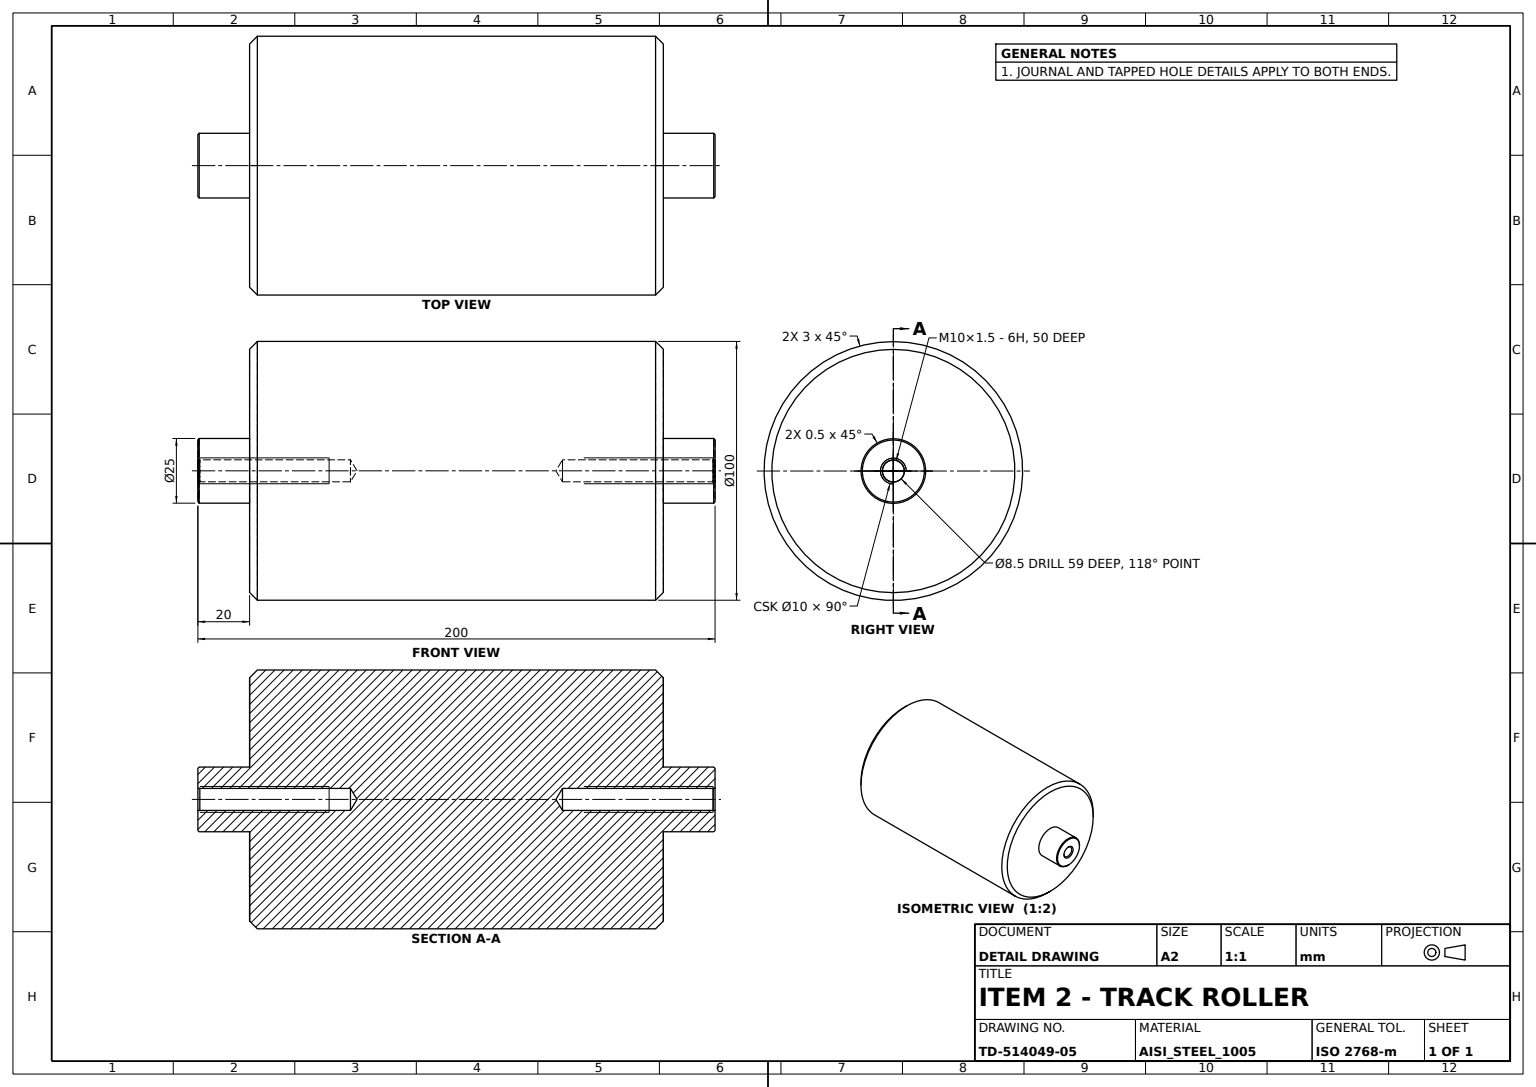
ISO-10303-21;
HEADER;
FILE_DESCRIPTION((''),'2;1');
FILE_NAME('','',(''),(''),'','','');
FILE_SCHEMA(('AUTOMOTIVE_DESIGN'));
ENDSEC;
DATA;
#1=APPLICATION_CONTEXT('');
#2=PRODUCT_CONTEXT('',#1,'mechanical');
#3=PRODUCT('','','',(#2));
#4=PRODUCT_DEFINITION_FORMATION('','',#3);
#5=PRODUCT_DEFINITION_CONTEXT('',#1,'design');
#6=PRODUCT_DEFINITION('','',#4,#5);
#7=PRODUCT_DEFINITION_SHAPE('','',#6);
#8=(LENGTH_UNIT()NAMED_UNIT(*)SI_UNIT(.MILLI.,.METRE.));
#9=(NAMED_UNIT(*)PLANE_ANGLE_UNIT()SI_UNIT($,.RADIAN.));
#10=(NAMED_UNIT(*)SI_UNIT($,.STERADIAN.)SOLID_ANGLE_UNIT());
#11=UNCERTAINTY_MEASURE_WITH_UNIT(LENGTH_MEASURE(0.005),#8,'distance_accuracy_value','');
#12=(GEOMETRIC_REPRESENTATION_CONTEXT(3)GLOBAL_UNCERTAINTY_ASSIGNED_CONTEXT((#11))GLOBAL_UNIT_ASSIGNED_CONTEXT((#8,#9,#10))REPRESENTATION_CONTEXT('',''));
#13=CARTESIAN_POINT('',(-12.,0.,100.));
#14=VERTEX_POINT('',#13);
#15=CARTESIAN_POINT('',(0.,0.,100.));
#16=DIRECTION('',(0.,0.,-1.));
#17=DIRECTION('',(-1.,0.,0.));
#18=AXIS2_PLACEMENT_3D('',#15,#16,#17);
#19=CIRCLE('',#18,12.);
#20=EDGE_CURVE('',#14,#14,#19,.F.);
#21=ORIENTED_EDGE('',*,*,#20,.T.);
#22=EDGE_LOOP('',(#21));
#23=FACE_BOUND('',#22,.T.);
#24=CARTESIAN_POINT('',(-5.,0.,100.));
#25=VERTEX_POINT('',#24);
#26=CIRCLE('',#18,5.);
#27=EDGE_CURVE('',#25,#25,#26,.T.);
#28=ORIENTED_EDGE('',*,*,#27,.T.);
#29=EDGE_LOOP('',(#28));
#30=FACE_BOUND('',#29,.T.);
#31=PLANE('',#18);
#32=ADVANCED_FACE('',(#23,#30),#31,.F.);
#33=CARTESIAN_POINT('',(4.25,0.,-41.));
#34=VERTEX_POINT('',#33);
#35=CARTESIAN_POINT('',(0.,0.,-41.));
#36=DIRECTION('',(0.,0.,1.));
#37=DIRECTION('',(1.,0.,0.));
#38=AXIS2_PLACEMENT_3D('',#35,#36,#37);
#39=CIRCLE('',#38,4.25);
#40=EDGE_CURVE('',#34,#34,#39,.T.);
#41=ORIENTED_EDGE('',*,*,#40,.F.);
#42=EDGE_LOOP('',(#41));
#43=FACE_BOUND('',#42,.T.);
#44=CARTESIAN_POINT('',(0.,0.,-38.446342));
#45=VERTEX_POINT('',#44);
#46=VERTEX_LOOP('',#45);
#47=FACE_BOUND('',#46,.T.);
#48=AXIS2_PLACEMENT_3D('',#35,#16,#17);
#49=CONICAL_SURFACE('',#48,4.25,1.029744259);
#50=ADVANCED_FACE('',(#43,#47),#49,.F.);
#51=CARTESIAN_POINT('',(-4.25,0.,99.25));
#52=VERTEX_POINT('',#51);
#53=CARTESIAN_POINT('',(0.,0.,99.25));
#54=AXIS2_PLACEMENT_3D('',#53,#16,#17);
#55=CIRCLE('',#54,4.25);
#56=EDGE_CURVE('',#52,#52,#55,.F.);
#57=ORIENTED_EDGE('',*,*,#56,.F.);
#58=EDGE_LOOP('',(#57));
#59=FACE_BOUND('',#58,.T.);
#60=ORIENTED_EDGE('',*,*,#27,.F.);
#61=EDGE_LOOP('',(#60));
#62=FACE_BOUND('',#61,.T.);
#63=AXIS2_PLACEMENT_3D('',#15,#36,#37);
#64=CONICAL_SURFACE('',#63,5.,0.785398163);
#65=ADVANCED_FACE('',(#59,#62),#64,.F.);
#66=CARTESIAN_POINT('',(-50.,0.,-77.));
#67=VERTEX_POINT('',#66);
#68=CARTESIAN_POINT('',(0.,0.,-77.));
#69=AXIS2_PLACEMENT_3D('',#68,#16,#17);
#70=CIRCLE('',#69,50.);
#71=EDGE_CURVE('',#67,#67,#70,.F.);
#72=ORIENTED_EDGE('',*,*,#71,.F.);
#73=EDGE_LOOP('',(#72));
#74=FACE_BOUND('',#73,.T.);
#75=CARTESIAN_POINT('',(-47.,0.,-80.));
#76=VERTEX_POINT('',#75);
#77=CARTESIAN_POINT('',(0.,0.,-80.));
#78=AXIS2_PLACEMENT_3D('',#77,#16,#17);
#79=CIRCLE('',#78,47.);
#80=EDGE_CURVE('',#76,#76,#79,.T.);
#81=ORIENTED_EDGE('',*,*,#80,.F.);
#82=EDGE_LOOP('',(#81));
#83=FACE_BOUND('',#82,.T.);
#84=AXIS2_PLACEMENT_3D('',#77,#36,#37);
#85=CONICAL_SURFACE('',#84,47.,0.785398163);
#86=ADVANCED_FACE('',(#74,#83),#85,.T.);
#87=CARTESIAN_POINT('',(-4.25,0.,41.));
#88=VERTEX_POINT('',#87);
#89=CARTESIAN_POINT('',(0.,0.,41.));
#90=AXIS2_PLACEMENT_3D('',#89,#16,#17);
#91=CIRCLE('',#90,4.25);
#92=EDGE_CURVE('',#88,#88,#91,.F.);
#93=ORIENTED_EDGE('',*,*,#92,.F.);
#94=EDGE_LOOP('',(#93));
#95=FACE_BOUND('',#94,.T.);
#96=ORIENTED_EDGE('',*,*,#56,.T.);
#97=EDGE_LOOP('',(#96));
#98=FACE_BOUND('',#97,.T.);
#99=CYLINDRICAL_SURFACE('',#18,4.25);
#100=ADVANCED_FACE('',(#95,#98),#99,.F.);
#101=CARTESIAN_POINT('',(-12.5,0.,-99.5));
#102=VERTEX_POINT('',#101);
#103=CARTESIAN_POINT('',(0.,0.,-99.5));
#104=AXIS2_PLACEMENT_3D('',#103,#16,#17);
#105=CIRCLE('',#104,12.5);
#106=EDGE_CURVE('',#102,#102,#105,.F.);
#107=ORIENTED_EDGE('',*,*,#106,.F.);
#108=EDGE_LOOP('',(#107));
#109=FACE_BOUND('',#108,.T.);
#110=CARTESIAN_POINT('',(-12.,0.,-100.));
#111=VERTEX_POINT('',#110);
#112=CARTESIAN_POINT('',(0.,0.,-100.));
#113=AXIS2_PLACEMENT_3D('',#112,#16,#17);
#114=CIRCLE('',#113,12.);
#115=EDGE_CURVE('',#111,#111,#114,.T.);
#116=ORIENTED_EDGE('',*,*,#115,.F.);
#117=EDGE_LOOP('',(#116));
#118=FACE_BOUND('',#117,.T.);
#119=AXIS2_PLACEMENT_3D('',#112,#36,#37);
#120=CONICAL_SURFACE('',#119,12.,0.785398163);
#121=ADVANCED_FACE('',(#109,#118),#120,.T.);
#122=ORIENTED_EDGE('',*,*,#80,.T.);
#123=EDGE_LOOP('',(#122));
#124=FACE_BOUND('',#123,.T.);
#125=CARTESIAN_POINT('',(12.5,0.,-80.));
#126=VERTEX_POINT('',#125);
#127=AXIS2_PLACEMENT_3D('',#77,#16,#37);
#128=CIRCLE('',#127,12.5);
#129=EDGE_CURVE('',#126,#126,#128,.T.);
#130=ORIENTED_EDGE('',*,*,#129,.F.);
#131=EDGE_LOOP('',(#130));
#132=FACE_BOUND('',#131,.T.);
#133=PLANE('',#78);
#134=ADVANCED_FACE('',(#124,#132),#133,.T.);
#135=CARTESIAN_POINT('',(-12.5,0.,99.5));
#136=VERTEX_POINT('',#135);
#137=CARTESIAN_POINT('',(0.,0.,99.5));
#138=AXIS2_PLACEMENT_3D('',#137,#16,#17);
#139=CIRCLE('',#138,12.5);
#140=EDGE_CURVE('',#136,#136,#139,.T.);
#141=ORIENTED_EDGE('',*,*,#140,.F.);
#142=EDGE_LOOP('',(#141));
#143=FACE_BOUND('',#142,.T.);
#144=ORIENTED_EDGE('',*,*,#20,.F.);
#145=EDGE_LOOP('',(#144));
#146=FACE_BOUND('',#145,.T.);
#147=CONICAL_SURFACE('',#138,12.5,0.785398163);
#148=ADVANCED_FACE('',(#143,#146),#147,.T.);
#149=ORIENTED_EDGE('',*,*,#106,.T.);
#150=EDGE_LOOP('',(#149));
#151=FACE_BOUND('',#150,.T.);
#152=ORIENTED_EDGE('',*,*,#129,.T.);
#153=EDGE_LOOP('',(#152));
#154=FACE_BOUND('',#153,.T.);
#155=CYLINDRICAL_SURFACE('',#119,12.5);
#156=ADVANCED_FACE('',(#151,#154),#155,.T.);
#157=CARTESIAN_POINT('',(-4.25,0.,-99.25));
#158=VERTEX_POINT('',#157);
#159=CARTESIAN_POINT('',(0.,0.,-99.25));
#160=AXIS2_PLACEMENT_3D('',#159,#16,#17);
#161=CIRCLE('',#160,4.25);
#162=EDGE_CURVE('',#158,#158,#161,.F.);
#163=ORIENTED_EDGE('',*,*,#162,.T.);
#164=EDGE_LOOP('',(#163));
#165=FACE_BOUND('',#164,.T.);
#166=CARTESIAN_POINT('',(-5.,0.,-100.));
#167=VERTEX_POINT('',#166);
#168=CIRCLE('',#113,5.);
#169=EDGE_CURVE('',#167,#167,#168,.F.);
#170=ORIENTED_EDGE('',*,*,#169,.F.);
#171=EDGE_LOOP('',(#170));
#172=FACE_BOUND('',#171,.T.);
#173=CONICAL_SURFACE('',#113,5.,0.785398163);
#174=ADVANCED_FACE('',(#165,#172),#173,.F.);
#175=CARTESIAN_POINT('',(-47.,0.,80.));
#176=VERTEX_POINT('',#175);
#177=CARTESIAN_POINT('',(0.,0.,80.));
#178=AXIS2_PLACEMENT_3D('',#177,#16,#17);
#179=CIRCLE('',#178,47.);
#180=EDGE_CURVE('',#176,#176,#179,.F.);
#181=ORIENTED_EDGE('',*,*,#180,.T.);
#182=EDGE_LOOP('',(#181));
#183=FACE_BOUND('',#182,.T.);
#184=CARTESIAN_POINT('',(12.5,0.,80.));
#185=VERTEX_POINT('',#184);
#186=AXIS2_PLACEMENT_3D('',#177,#16,#37);
#187=CIRCLE('',#186,12.5);
#188=EDGE_CURVE('',#185,#185,#187,.T.);
#189=ORIENTED_EDGE('',*,*,#188,.T.);
#190=EDGE_LOOP('',(#189));
#191=FACE_BOUND('',#190,.T.);
#192=PLANE('',#178);
#193=ADVANCED_FACE('',(#183,#191),#192,.F.);
#194=ORIENTED_EDGE('',*,*,#92,.T.);
#195=EDGE_LOOP('',(#194));
#196=FACE_BOUND('',#195,.T.);
#197=CARTESIAN_POINT('',(0.,0.,38.446342));
#198=VERTEX_POINT('',#197);
#199=VERTEX_LOOP('',#198);
#200=FACE_BOUND('',#199,.T.);
#201=AXIS2_PLACEMENT_3D('',#89,#36,#37);
#202=CONICAL_SURFACE('',#201,4.25,1.029744259);
#203=ADVANCED_FACE('',(#196,#200),#202,.F.);
#204=ORIENTED_EDGE('',*,*,#169,.T.);
#205=EDGE_LOOP('',(#204));
#206=FACE_BOUND('',#205,.T.);
#207=ORIENTED_EDGE('',*,*,#115,.T.);
#208=EDGE_LOOP('',(#207));
#209=FACE_BOUND('',#208,.T.);
#210=PLANE('',#113);
#211=ADVANCED_FACE('',(#206,#209),#210,.T.);
#212=ORIENTED_EDGE('',*,*,#188,.F.);
#213=EDGE_LOOP('',(#212));
#214=FACE_BOUND('',#213,.T.);
#215=ORIENTED_EDGE('',*,*,#140,.T.);
#216=EDGE_LOOP('',(#215));
#217=FACE_BOUND('',#216,.T.);
#218=CYLINDRICAL_SURFACE('',#18,12.5);
#219=ADVANCED_FACE('',(#214,#217),#218,.T.);
#220=ORIENTED_EDGE('',*,*,#162,.F.);
#221=EDGE_LOOP('',(#220));
#222=FACE_BOUND('',#221,.T.);
#223=ORIENTED_EDGE('',*,*,#40,.T.);
#224=EDGE_LOOP('',(#223));
#225=FACE_BOUND('',#224,.T.);
#226=CYLINDRICAL_SURFACE('',#119,4.25);
#227=ADVANCED_FACE('',(#222,#225),#226,.F.);
#228=ORIENTED_EDGE('',*,*,#71,.T.);
#229=EDGE_LOOP('',(#228));
#230=FACE_BOUND('',#229,.T.);
#231=CARTESIAN_POINT('',(-50.,0.,77.));
#232=VERTEX_POINT('',#231);
#233=CARTESIAN_POINT('',(0.,0.,77.));
#234=AXIS2_PLACEMENT_3D('',#233,#16,#17);
#235=CIRCLE('',#234,50.);
#236=EDGE_CURVE('',#232,#232,#235,.T.);
#237=ORIENTED_EDGE('',*,*,#236,.T.);
#238=EDGE_LOOP('',(#237));
#239=FACE_BOUND('',#238,.T.);
#240=CYLINDRICAL_SURFACE('',#178,50.);
#241=ADVANCED_FACE('',(#230,#239),#240,.T.);
#242=ORIENTED_EDGE('',*,*,#180,.F.);
#243=EDGE_LOOP('',(#242));
#244=FACE_BOUND('',#243,.T.);
#245=ORIENTED_EDGE('',*,*,#236,.F.);
#246=EDGE_LOOP('',(#245));
#247=FACE_BOUND('',#246,.T.);
#248=CONICAL_SURFACE('',#234,50.,0.785398163);
#249=ADVANCED_FACE('',(#244,#247),#248,.T.);
#250=CLOSED_SHELL('',(#32,#50,#65,#86,#100,#121,#134,#148,#156,#174,#193,#203,#211,#219,#227,#241,#249));
#251=MANIFOLD_SOLID_BREP('',#250);
#252=ADVANCED_BREP_SHAPE_REPRESENTATION('',(#251),#12);
#253=SHAPE_DEFINITION_REPRESENTATION(#7,#252);
ENDSEC;
END-ISO-10303-21;
